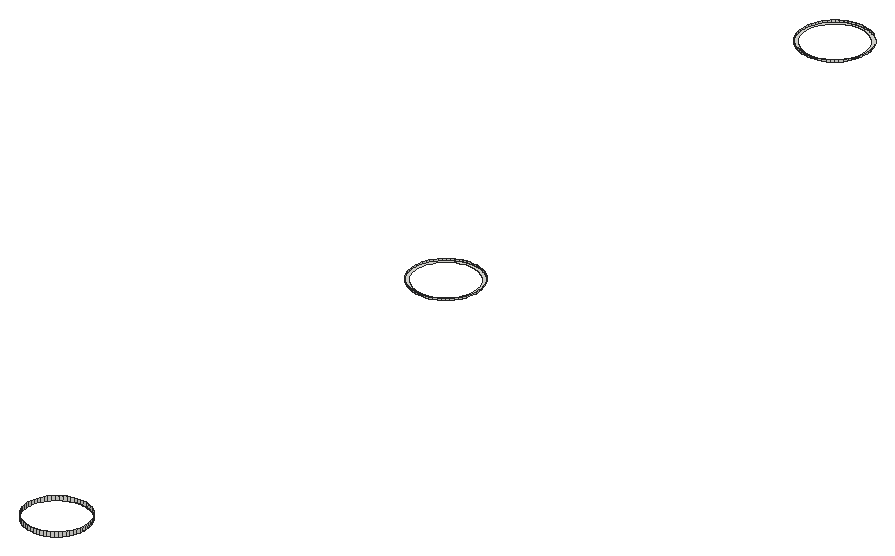
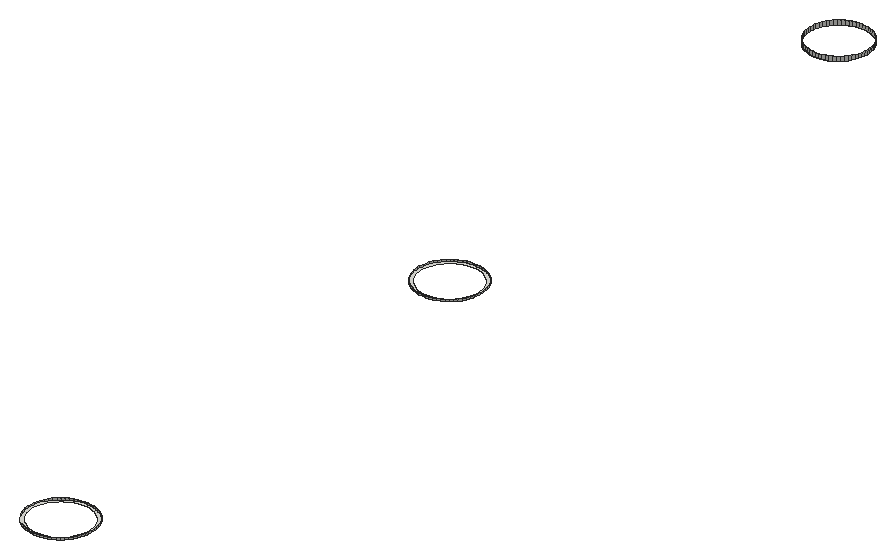
# SketchUp Ruby script. Lengths in inches.
U = 1.inch
M = Sketchup.active_model
def pt(a) = Geom::Point3d.new(a.map { |v| v * U })
def face(e, loops, mat)
  f = e.add_face(loops[0].map { |a| pt(a) })
  loops[1..].each { |l| e.add_face(l.map { |a| pt(a) }).erase! }
  f.material = f.back_material = mat if mat
  f
end
# faces: each face lists its corners as indices into pts; further lists are holes
def faces(e, pts, list, mat = nil) = list.each { |f| face(e, (f[0].is_a?(Array) ? f : [f]).map { |l| l.map { |i| pts[i] } }, mat) }
# xy, xz, yz: faces in a plane at the given z, y or x. An outline is a flat list of corners, or four numbers for a rectangle; further outlines are holes
def ring(l) = l.size == 4 ? [[l[0], l[1]], [l[2], l[1]], [l[2], l[3]], [l[0], l[3]]] : l.each_slice(2).to_a
def flat(e, list, mat, &to3) = list.each { |f| face(e, (f[0].is_a?(Array) ? f : [f]).map { |l| ring(l).map { |u, v| to3.(u, v) } }, mat) }
def xy(e, z, list, mat = nil) = flat(e, list, mat) { |x, y| [x, y, z] }
def xz(e, y, list, mat = nil) = flat(e, list, mat) { |x, z| [x, y, z] }
def yz(e, x, list, mat = nil) = flat(e, list, mat) { |y, z| [x, y, z] }
def lines(e, pts, list) = list.each { |a, b| e.add_line(pt(pts[a]), pt(pts[b])) }
# prism: a flat outline (further loops are holes) pulled along v
def prism(e, loops, v, mat = nil)
  f = face(e, loops, mat); d = Geom::Vector3d.new(v.map { |x| x * U })
  f.pushpull(f.normal.samedirection?(d) ? d.length : -d.length)
end
def box(e, o, s, mat = nil) = prism(e, [[o, [o[0] + s[0], o[1], o[2]], [o[0] + s[0], o[1] + s[1], o[2]], [o[0], o[1] + s[1], o[2]]]], [0, 0, s[2]], mat)
def at(x, y, z, deg = 0) = Geom::Transformation.translation(pt([x, y, z])) * Geom::Transformation.rotation(ORIGIN, Z_AXIS, deg.degrees)
def axes(o, x, y, z) = Geom::Transformation.new([*x, 0, *y, 0, *z, 0, *pt(o).to_a, 1])
def part(name) = M.definitions.add(name)
# library, detail: a bought-in or finely detailed component or shape, given as its bounding box
def library(name, o, s) = part(name).tap { |d| box(d.entities, o, s) }
def detail(e, o, s) = box(e.add_group.entities, o, s)
def put(e, d, t, mat = nil) = e.add_instance(d, t).tap { |i| i.material = mat if mat }
def group(e, t, mat = nil) = e.add_group.tap { |g| g.transformation = t; g.material = mat if mat }.entities
root = M.entities
xy(root,113.9,[[18.649,8.139,18.682,8.344,18.671,8.241],[18.682,8.344,18.695,8.552,18.694,8.448],[18.695,8.552,18.685,8.76,18.695,8.657],[18.685,8.76,18.653,8.966,18.675,8.864],[18.653,8.966,18.601,9.168,18.632,9.068],
  [18.601,9.168,18.527,9.363,18.569,9.267],[18.527,9.363,18.434,9.549,18.485,9.458],[18.434,9.549,18.321,9.724,18.382,9.64],[18.321,9.724,18.191,9.887,18.261,9.809],[18.191,9.887,18.045,10.035,18.122,9.965],
  [18.045,10.035,17.884,10.167,17.968,10.105],[17.884,10.167,17.71,10.282,17.8,10.229],[17.71,10.282,17.525,10.377,17.62,10.334],[17.525,10.377,17.331,10.453,17.43,10.42],[15.906,10.387,16.001,10.429,16.101,10.46],
  [17.331,10.453,17.13,10.508,17.232,10.486],[16.101,10.46,16.2,10.492,16.302,10.513],[17.13,10.508,16.924,10.542,17.028,10.53],[16.302,10.513,16.404,10.534,16.508,10.544],[16.924,10.542,16.716,10.554,16.82,10.553],
  [16.508,10.544,16.612,10.555,16.716,10.554],[[16.806,39.72,16.577,39.722,16.349,39.747,16.125,39.796,15.907,39.868,15.697,39.963,15.499,40.079,15.315,40.215,15.145,40.369,14.992,40.541,14.858,40.727,14.745,40.927,14.653,41.137,14.583,41.356,14.537,41.581,14.514,41.809,14.515,42.039,14.541,42.267,14.59,42.491,14.662,42.709,14.757,42.918,14.872,43.116,15.008,43.301,15.163,43.471,15.335,43.623,15.521,43.757,15.72,43.871,15.931,43.963,16.149,44.032,16.374,44.079,16.603,44.101,16.832,44.1,17.06,44.075,17.284,44.026,17.502,43.953,17.711,43.859,17.91,43.743,18.094,43.607,18.264,43.452,18.417,43.281,18.551,43.094,18.664,42.895,18.756,42.685,18.826,42.466,18.872,42.241,18.895,42.013,18.894,41.783,18.868,41.555,18.819,41.331,18.747,41.113,18.652,40.904,18.537,40.706,18.4,40.521,18.246,40.351,18.074,40.199,17.888,40.065,17.689,39.951,17.478,39.859,17.26,39.79,17.035,39.743],[16.797,39.92,17.005,39.941,17.209,39.983,17.408,40.046,17.599,40.13,17.78,40.233,17.949,40.355,18.105,40.494,18.246,40.648,18.369,40.816,18.475,40.996,18.561,41.186,18.626,41.384,18.671,41.588,18.694,41.795,18.695,42.004,18.675,42.211,18.632,42.415,18.569,42.614,18.485,42.805,18.382,42.986,18.261,43.156,18.122,43.312,17.968,43.452,17.8,43.576,17.62,43.681,17.43,43.767,17.232,43.833,17.028,43.877,16.82,43.9,16.612,43.902,16.404,43.881,16.2,43.839,16.001,43.776,15.81,43.692,15.629,43.589,15.459,43.467,15.304,43.328,15.163,43.174,15.04,43.006,14.934,42.826,14.848,42.636,14.783,42.438,14.738,42.234,14.715,42.027,14.714,41.818,14.734,41.611,14.777,41.406,14.84,41.208,14.924,41.017,15.027,40.835,15.148,40.666,15.287,40.51,15.441,40.37,15.609,40.246,15.789,40.141,15.979,40.055,16.177,39.989,16.381,39.944,16.588,39.921]],[[16.806,73.067,16.577,73.069,16.349,73.094,16.125,73.143,15.907,73.215,15.697,73.31,15.499,73.426,15.315,73.562,15.145,73.716,14.992,73.888,14.858,74.074,14.745,74.274,14.653,74.484,14.583,74.703,14.537,74.928,14.514,75.156,14.515,75.385,14.541,75.614,14.59,75.838,14.662,76.056,14.757,76.265,14.872,76.463,15.008,76.648,15.163,76.817,15.335,76.97,15.521,77.104,15.72,77.217,15.931,77.31,16.149,77.379,16.374,77.426,16.603,77.448,16.832,77.447,17.06,77.422,17.284,77.373,17.502,77.3,17.711,77.206,17.91,77.09,18.094,76.954,18.264,76.799,18.417,76.628,18.551,76.441,18.664,76.242,18.756,76.032,18.826,75.813,18.872,75.588,18.895,75.36,18.894,75.13,18.868,74.902,18.819,74.678,18.747,74.46,18.652,74.251,18.537,74.053,18.4,73.868,18.246,73.698,18.074,73.546,17.888,73.412,17.689,73.298,17.478,73.206,17.26,73.136,17.035,73.09],[16.797,73.267,17.005,73.288,17.209,73.33,17.408,73.393,17.599,73.477,17.78,73.58,17.949,73.702,18.105,73.84,18.246,73.995,18.369,74.163,18.475,74.343,18.561,74.533,18.626,74.731,18.671,74.935,18.694,75.142,18.695,75.35,18.675,75.558,18.632,75.762,18.569,75.961,18.485,76.152,18.382,76.333,18.261,76.503,18.122,76.659,17.968,76.799,17.8,76.923,17.62,77.028,17.43,77.114,17.232,77.18,17.028,77.224,16.82,77.247,16.612,77.249,16.404,77.228,16.2,77.186,16.001,77.122,15.81,77.039,15.629,76.936,15.459,76.814,15.304,76.675,15.163,76.521,15.04,76.353,14.934,76.173,14.848,75.983,14.783,75.785,14.738,75.581,14.715,75.374,14.714,75.165,14.734,74.958,14.777,74.753,14.84,74.555,14.924,74.364,15.027,74.182,15.148,74.013,15.287,73.857,15.441,73.717,15.609,73.593,15.789,73.488,15.979,73.402,16.177,73.336,16.381,73.291,16.588,73.268]]])
p = [[16.279,6.62,113.9],[16.078,6.675,113.9],[16.078,6.675,114.189],[16.279,6.62,114.189],[16.485,6.586,113.9],[16.485,6.586,114.189],
  [16.693,6.574,113.9],[16.693,6.574,114.189],[16.901,6.584,113.9],[16.901,6.584,114.189],[17.107,6.615,113.9],[17.107,6.615,114.189],
  [17.308,6.668,113.9],[17.308,6.668,114.189],[15.884,6.751,113.9],[15.884,6.751,114.189],[17.503,6.741,113.9],[17.503,6.741,114.189],
  [17.689,6.835,113.9],[17.689,6.835,114.189],[15.699,6.846,113.9],[15.525,6.961,113.9],[15.525,6.961,114.189],[15.699,6.846,114.189],
  [17.865,6.947,113.9],[17.865,6.947,114.189],[18.027,7.077,113.9],[18.027,7.077,114.189],[15.364,7.093,113.9],[15.364,7.093,114.189],
  [15.218,7.241,113.9],[15.218,7.241,114.189],[18.176,7.224,113.9],[18.176,7.224,114.189],[15.088,7.404,113.9],[15.088,7.404,114.189],
  [18.308,7.385,113.9],[18.308,7.385,114.189],[14.975,7.579,113.9],[14.975,7.579,114.189],[18.422,7.559,113.9],[18.422,7.559,114.189],
  [14.882,7.765,113.9],[14.882,7.765,114.189],[18.518,7.744,113.9],[18.518,7.744,114.189],[18.594,7.938,113.9],[18.594,7.938,114.189],
  [14.808,7.96,113.9],[14.808,7.96,114.189],[18.649,8.139,113.9],[18.649,8.139,114.189],[14.755,8.162,113.9],[14.755,8.162,114.189],
  [18.682,8.344,113.9],[18.682,8.344,114.189],[14.724,8.368,113.9],[14.724,8.368,114.189],[18.695,8.552,113.9],[18.695,8.552,114.189],
  [14.714,8.576,113.9],[14.714,8.576,114.189],[14.727,8.784,113.9],[14.727,8.784,114.189],[18.685,8.76,113.9],[18.685,8.76,114.189],
  [14.76,8.989,113.9],[14.76,8.989,114.189],[18.653,8.966,113.9],[18.653,8.966,114.189],[14.815,9.19,113.9],[14.815,9.19,114.189],
  [18.601,9.168,113.9],[18.601,9.168,114.189],[14.891,9.384,113.9],[14.891,9.384,114.189],[18.527,9.363,113.9],[18.527,9.363,114.189],
  [14.987,9.569,113.9],[14.987,9.569,114.189],[18.434,9.549,113.9],[18.434,9.549,114.189],[18.321,9.724,113.9],[18.321,9.724,114.189],
  [15.101,9.743,113.9],[15.101,9.743,114.189],[15.233,9.904,113.9],[15.233,9.904,114.189],[18.191,9.887,113.9],[18.191,9.887,114.189],
  [15.382,10.051,113.9],[15.382,10.051,114.189],[18.045,10.035,113.9],[18.045,10.035,114.189],[17.884,10.167,113.9],[17.884,10.167,114.189],
  [15.544,10.181,113.9],[15.544,10.181,114.189],[15.72,10.293,113.9],[15.72,10.293,114.189],[17.71,10.282,113.9],[17.71,10.282,114.189],
  [15.906,10.387,113.9],[15.906,10.387,114.189],[17.525,10.377,113.9],[17.525,10.377,114.189],[16.101,10.46,113.9],[16.101,10.46,114.189],
  [17.331,10.453,113.9],[17.331,10.453,114.189],[16.302,10.513,113.9],[16.302,10.513,114.189],[16.508,10.544,113.9],[16.508,10.544,114.189],
  [16.716,10.554,113.9],[16.716,10.554,114.189],[16.924,10.542,113.9],[16.924,10.542,114.189],[17.13,10.508,113.9],[17.13,10.508,114.189],
  [16.349,39.747,114],[16.125,39.796,114],[16.125,39.796,113.9],[16.349,39.747,113.9],[16.577,39.722,114],[16.577,39.722,113.9],
  [16.806,39.72,114],[16.806,39.72,113.9],[17.035,39.743,114],[17.035,39.743,113.9],[17.26,39.79,114],[17.26,39.79,113.9],
  [15.907,39.868,114],[15.907,39.868,113.9],[17.478,39.859,114],[17.478,39.859,113.9],[15.697,39.963,114],[15.697,39.963,113.9],
  [17.689,39.951,114],[17.689,39.951,113.9],[15.499,40.079,114],[15.499,40.079,113.9],[17.888,40.065,114],[17.888,40.065,113.9],
  [15.315,40.215,114],[15.315,40.215,113.9],[18.074,40.199,114],[18.074,40.199,113.9],[15.145,40.369,114],[15.145,40.369,113.9],
  [18.246,40.351,114],[18.246,40.351,113.9],[14.992,40.541,114],[14.992,40.541,113.9],[18.4,40.521,114],[18.4,40.521,113.9],
  [14.858,40.727,114],[14.858,40.727,113.9],[18.537,40.706,114],[18.537,40.706,113.9],[14.745,40.927,114],[14.745,40.927,113.9],
  [18.652,40.904,114],[18.652,40.904,113.9],[14.653,41.137,114],[14.653,41.137,113.9],[18.747,41.113,114],[18.747,41.113,113.9],
  [14.583,41.356,114],[14.583,41.356,113.9],[18.819,41.331,114],[18.819,41.331,113.9],[18.868,41.555,114],[18.868,41.555,113.9],
  [14.537,41.581,114],[14.537,41.581,113.9],[14.514,41.809,114],[14.514,41.809,113.9],[18.894,41.783,114],[18.894,41.783,113.9],
  [14.515,42.039,114],[14.515,42.039,113.9],[18.895,42.013,114],[18.895,42.013,113.9],[14.541,42.267,114],[14.541,42.267,113.9],
  [18.872,42.241,114],[18.872,42.241,113.9],[18.826,42.466,114],[18.826,42.466,113.9],[14.59,42.491,114],[14.59,42.491,113.9],
  [14.662,42.709,114],[14.662,42.709,113.9],[18.756,42.685,114],[18.756,42.685,113.9],[14.757,42.918,114],[14.757,42.918,113.9],
  [18.664,42.895,114],[18.664,42.895,113.9],[14.872,43.116,114],[14.872,43.116,113.9],[18.551,43.094,114],[18.551,43.094,113.9],
  [15.008,43.301,114],[15.008,43.301,113.9],[18.417,43.281,114],[18.417,43.281,113.9],[15.163,43.471,114],[15.163,43.471,113.9],
  [18.264,43.452,114],[18.264,43.452,113.9],[15.335,43.623,114],[15.335,43.623,113.9],[18.094,43.607,114],[18.094,43.607,113.9],
  [15.521,43.757,114],[15.521,43.757,113.9],[17.91,43.743,114],[17.91,43.743,113.9],[17.711,43.859,114],[17.711,43.859,113.9],
  [15.72,43.871,114],[15.72,43.871,113.9],[15.931,43.963,114],[15.931,43.963,113.9],[17.502,43.953,114],[17.502,43.953,113.9],
  [16.149,44.032,114],[16.149,44.032,113.9],[16.374,44.079,114],[16.374,44.079,113.9],[17.06,44.075,114],[17.284,44.026,114],
  [17.284,44.026,113.9],[17.06,44.075,113.9],[16.603,44.101,114],[16.603,44.101,113.9],[16.832,44.1,114],[16.832,44.1,113.9],
  [16.125,73.143,114],[15.907,73.215,114],[15.907,73.215,113.9],[16.125,73.143,113.9],[16.349,73.094,114],[16.349,73.094,113.9],
  [16.577,73.069,114],[16.577,73.069,113.9],[16.806,73.067,114],[16.806,73.067,113.9],[17.035,73.09,114],[17.035,73.09,113.9],
  [17.26,73.136,114],[17.26,73.136,113.9],[17.478,73.206,114],[17.478,73.206,113.9],[15.697,73.31,114],[15.697,73.31,113.9],
  [17.689,73.298,114],[17.689,73.298,113.9],[15.499,73.426,114],[15.499,73.426,113.9],[17.888,73.412,114],[17.888,73.412,113.9],
  [15.315,73.562,114],[15.315,73.562,113.9],[18.074,73.546,114],[18.074,73.546,113.9],[18.246,73.698,114],[18.246,73.698,113.9],
  [15.145,73.716,114],[15.145,73.716,113.9],[14.992,73.888,114],[14.992,73.888,113.9],[18.4,73.868,114],[18.4,73.868,113.9],
  [14.858,74.074,114],[14.858,74.074,113.9],[18.537,74.053,114],[18.537,74.053,113.9],[14.745,74.274,114],[14.745,74.274,113.9],
  [18.652,74.251,114],[18.652,74.251,113.9],[14.653,74.484,114],[14.653,74.484,113.9],[18.747,74.46,114],[18.747,74.46,113.9],
  [14.583,74.703,114],[14.583,74.703,113.9],[18.819,74.678,114],[18.819,74.678,113.9],[14.537,74.928,114],[14.537,74.928,113.9],
  [18.868,74.902,114],[18.868,74.902,113.9],[14.514,75.156,114],[14.514,75.156,113.9],[18.894,75.13,114],[18.894,75.13,113.9],
  [18.895,75.36,114],[18.895,75.36,113.9],[14.515,75.385,114],[14.515,75.385,113.9],[14.541,75.614,114],[14.541,75.614,113.9],
  [18.872,75.588,114],[18.872,75.588,113.9],[14.59,75.838,114],[14.59,75.838,113.9],[18.826,75.813,114],[18.826,75.813,113.9],
  [14.662,76.056,114],[14.662,76.056,113.9],[18.756,76.032,114],[18.756,76.032,113.9],[18.664,76.242,114],[18.664,76.242,113.9],
  [14.757,76.265,114],[14.757,76.265,113.9],[14.872,76.463,114],[14.872,76.463,113.9],[15.008,76.648,114],[15.008,76.648,113.9],
  [15.163,76.817,114],[15.163,76.817,113.9],[15.335,76.97,114],[15.335,76.97,113.9],[15.521,77.104,114],[15.521,77.104,113.9],
  [15.72,77.217,114],[15.72,77.217,113.9],[17.711,77.206,114],[17.91,77.09,114],[17.91,77.09,113.9],[17.711,77.206,113.9],
  [15.931,77.31,114],[15.931,77.31,113.9],[17.502,77.3,114],[17.502,77.3,113.9],[16.149,77.379,114],[16.149,77.379,113.9],
  [17.284,77.373,114],[17.284,77.373,113.9],[16.374,77.426,114],[16.374,77.426,113.9],[16.603,77.448,114],[16.603,77.448,113.9],
  [16.832,77.447,114],[16.832,77.447,113.9],[17.06,77.422,114],[17.06,77.422,113.9]]
faces(root,p,[[0,1,2,3],[4,0,3,5],[6,4,5,7],[8,6,7,9],[10,8,9,11],[12,10,11,13],[1,14,15,2],[16,12,13,17],
  [18,16,17,19],[20,21,22,23],[14,20,23,15],[24,18,19,25],[26,24,25,27],[21,28,29,22],[28,30,31,29],[32,26,27,33],
  [30,34,35,31],[36,32,33,37],[34,38,39,35],[40,36,37,41],[38,42,43,39],[44,40,41,45],[46,44,45,47],[42,48,49,43],
  [50,46,47,51],[48,52,53,49],[54,50,51,55],[52,56,57,53],[58,54,55,59],[56,60,61,57],[60,62,63,61],[64,58,59,65],
  [62,66,67,63],[68,64,65,69],[66,70,71,67],[72,68,69,73],[70,74,75,71],[76,72,73,77],[74,78,79,75],[80,76,77,81],
  [82,80,81,83],[78,84,85,79],[84,86,87,85],[88,82,83,89],[86,90,91,87],[92,88,89,93],[94,92,93,95],[90,96,97,91],
  [96,98,99,97],[100,94,95,101],[98,102,103,99],[104,100,101,105],[102,106,107,103],[108,104,105,109],[106,110,111,107],[110,112,113,111],
  [112,114,115,113],[114,116,117,115],[116,118,119,117],[118,108,109,119],[120,121,122,123],[124,120,123,125],[126,124,125,127],[128,126,127,129],
  [130,128,129,131],[121,132,133,122],[134,130,131,135],[132,136,137,133],[138,134,135,139],[136,140,141,137],[142,138,139,143],[140,144,145,141],
  [146,142,143,147],[144,148,149,145],[150,146,147,151],[148,152,153,149],[154,150,151,155],[152,156,157,153],[158,154,155,159],[156,160,161,157],
  [162,158,159,163],[160,164,165,161],[166,162,163,167],[164,168,169,165],[170,166,167,171],[172,170,171,173],[168,174,175,169],[174,176,177,175],
  [178,172,173,179],[176,180,181,177],[182,178,179,183],[180,184,185,181],[186,182,183,187],[188,186,187,189],[184,190,191,185],[190,192,193,191],
  [194,188,189,195],[192,196,197,193],[198,194,195,199],[196,200,201,197],[202,198,199,203],[200,204,205,201],[206,202,203,207],[204,208,209,205],
  [210,206,207,211],[208,212,213,209],[214,210,211,215],[212,216,217,213],[218,214,215,219],[220,218,219,221],[216,222,223,217],[222,224,225,223],
  [226,220,221,227],[224,228,229,225],[228,230,231,229],[232,233,234,235],[233,226,227,234],[230,236,237,231],[236,238,239,237],[238,232,235,239],
  [240,241,242,243],[244,240,243,245],[246,244,245,247],[248,246,247,249],[250,248,249,251],[252,250,251,253],[254,252,253,255],[241,256,257,242],
  [258,254,255,259],[256,260,261,257],[262,258,259,263],[260,264,265,261],[266,262,263,267],[268,266,267,269],[264,270,271,265],[270,272,273,271],
  [274,268,269,275],[272,276,277,273],[278,274,275,279],[276,280,281,277],[282,278,279,283],[280,284,285,281],[286,282,283,287],[284,288,289,285],
  [290,286,287,291],[288,292,293,289],[294,290,291,295],[292,296,297,293],[298,294,295,299],[300,298,299,301],[296,302,303,297],[302,304,305,303],
  [306,300,301,307],[304,308,309,305],[310,306,307,311],[308,312,313,309],[314,310,311,315],[316,314,315,317],[312,318,319,313],[318,320,321,319],
  [320,322,323,321],[322,324,325,323],[324,326,327,325],[326,328,329,327],[328,330,331,329],[332,333,334,335],[330,336,337,331],[338,332,335,339],
  [336,340,341,337],[342,338,339,343],[340,344,345,341],[344,346,347,345],[346,348,349,347],[348,350,351,349],[350,342,343,351]])
